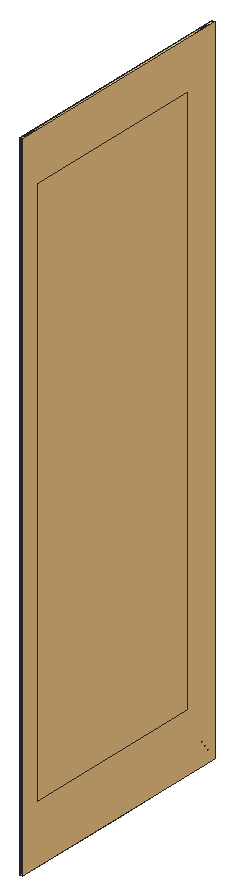
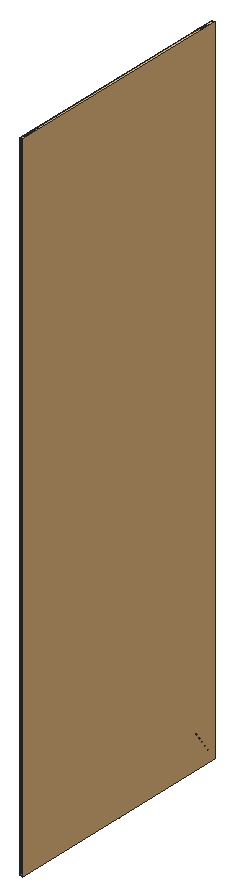
# SketchUp Ruby script. Lengths in inches.
U = 1.inch
M = Sketchup.active_model
def pt(a) = Geom::Point3d.new(a.map { |v| v * U })
def face(e, loops, mat)
  f = e.add_face(loops[0].map { |a| pt(a) })
  loops[1..].each { |l| e.add_face(l.map { |a| pt(a) }).erase! }
  f.material = f.back_material = mat if mat
  f
end
# faces: each face lists its corners as indices into pts; further lists are holes
def faces(e, pts, list, mat = nil) = list.each { |f| face(e, (f[0].is_a?(Array) ? f : [f]).map { |l| l.map { |i| pts[i] } }, mat) }
# xy, xz, yz: faces in a plane at the given z, y or x. An outline is a flat list of corners, or four numbers for a rectangle; further outlines are holes
def ring(l) = l.size == 4 ? [[l[0], l[1]], [l[2], l[1]], [l[2], l[3]], [l[0], l[3]]] : l.each_slice(2).to_a
def flat(e, list, mat, &to3) = list.each { |f| face(e, (f[0].is_a?(Array) ? f : [f]).map { |l| ring(l).map { |u, v| to3.(u, v) } }, mat) }
def xy(e, z, list, mat = nil) = flat(e, list, mat) { |x, y| [x, y, z] }
def xz(e, y, list, mat = nil) = flat(e, list, mat) { |x, z| [x, y, z] }
def yz(e, x, list, mat = nil) = flat(e, list, mat) { |y, z| [x, y, z] }
def lines(e, pts, list) = list.each { |a, b| e.add_line(pt(pts[a]), pt(pts[b])) }
# prism: a flat outline (further loops are holes) pulled along v
def prism(e, loops, v, mat = nil)
  f = face(e, loops, mat); d = Geom::Vector3d.new(v.map { |x| x * U })
  f.pushpull(f.normal.samedirection?(d) ? d.length : -d.length)
end
def box(e, o, s, mat = nil) = prism(e, [[o, [o[0] + s[0], o[1], o[2]], [o[0] + s[0], o[1] + s[1], o[2]], [o[0], o[1] + s[1], o[2]]]], [0, 0, s[2]], mat)
def at(x, y, z, deg = 0) = Geom::Transformation.translation(pt([x, y, z])) * Geom::Transformation.rotation(ORIGIN, Z_AXIS, deg.degrees)
def axes(o, x, y, z) = Geom::Transformation.new([*x, 0, *y, 0, *z, 0, *pt(o).to_a, 1])
def part(name) = M.definitions.add(name)
# library, detail: a bought-in or finely detailed component or shape, given as its bounding box
def library(name, o, s) = part(name).tap { |d| box(d.entities, o, s) }
def detail(e, o, s) = box(e.add_group.entities, o, s)
def put(e, d, t, mat = nil) = e.add_instance(d, t).tap { |i| i.material = mat if mat }
def group(e, t, mat = nil) = e.add_group.tap { |g| g.transformation = t; g.material = mat if mat }.entities
root = M.entities
M.materials.add("Material \#0").color = [86, 53, 35]
M.materials.add("Material \#1").color = [140, 140, 140]
c1 = part("3DGeom~8_Defintion")
xz(c1.entities,-471.94,[[458.125,-17.29,459.53,-16.11,457.73,-17.15],[458.125,-17.29,458.54,-17.29,459.53,-16.11],[458.54,-17.29,458.93,-17.15,459.53,-16.11],[457.73,-17.15,459.53,-16.11,457.42,-16.88],[458.93,-17.15,459.25,-16.88,459.53,-16.11],
  [457.42,-16.88,459.53,-16.11,457.21,-16.52],[459.25,-16.88,459.46,-16.52,459.53,-16.11],[457.21,-16.52,459.53,-16.11,457.14,-16.11],[457.14,-16.11,459.53,-16.11,457.21,-15.7],[459.53,-16.11,457.42,-15.34,457.21,-15.7],
  [459.53,-16.11,457.73,-15.07,457.42,-15.34],[459.53,-16.11,458.125,-14.93,457.73,-15.07],[459.53,-16.11,458.54,-14.93,458.125,-14.93],[459.53,-16.11,458.93,-15.07,458.54,-14.93],[459.53,-16.11,459.25,-15.34,458.93,-15.07],
  [459.53,-16.11,459.46,-15.7,459.25,-15.34]],"Material \#1")
xz(c1.entities,-416.39,[[458.125,-17.29,457.73,-17.15,459.53,-16.11],[458.125,-17.29,459.53,-16.11,458.54,-17.29],[458.54,-17.29,459.53,-16.11,458.93,-17.15],[457.73,-17.15,457.42,-16.88,459.53,-16.11],[458.93,-17.15,459.53,-16.11,459.25,-16.88],
  [457.42,-16.88,457.21,-16.52,459.53,-16.11],[459.25,-16.88,459.53,-16.11,459.46,-16.52],[457.21,-16.52,457.14,-16.11,459.53,-16.11],[457.14,-16.11,457.21,-15.7,459.53,-16.11],[459.53,-16.11,457.21,-15.7,457.42,-15.34],
  [459.53,-16.11,457.42,-15.34,457.73,-15.07],[459.53,-16.11,457.73,-15.07,458.125,-14.93],[459.53,-16.11,458.125,-14.93,458.54,-14.93],[459.53,-16.11,458.54,-14.93,458.93,-15.07],[459.53,-16.11,458.93,-15.07,459.25,-15.34],
  [459.53,-16.11,459.25,-15.34,459.46,-15.7]],"Material \#1")
xz(c1.entities,-27.5,[[458.125,-17.29,459.53,-16.11,457.73,-17.15],[458.125,-17.29,458.54,-17.29,459.53,-16.11],[458.54,-17.29,458.93,-17.15,459.53,-16.11],[457.73,-17.15,459.53,-16.11,457.42,-16.88],[458.93,-17.15,459.25,-16.88,459.53,-16.11],
  [457.42,-16.88,459.53,-16.11,457.21,-16.52],[459.25,-16.88,459.46,-16.52,459.53,-16.11],[457.21,-16.52,459.53,-16.11,457.14,-16.11],[457.14,-16.11,459.53,-16.11,457.21,-15.7],[459.53,-16.11,457.42,-15.34,457.21,-15.7],
  [459.53,-16.11,457.73,-15.07,457.42,-15.34],[459.53,-16.11,458.125,-14.93,457.73,-15.07],[459.53,-16.11,458.54,-14.93,458.125,-14.93],[459.53,-16.11,458.93,-15.07,458.54,-14.93],[459.53,-16.11,459.25,-15.34,458.93,-15.07],
  [459.53,-16.11,459.46,-15.7,459.25,-15.34]],"Material \#1")
xz(c1.entities,28.06,[[458.125,-17.29,457.73,-17.15,459.53,-16.11],[458.125,-17.29,459.53,-16.11,458.54,-17.29],[458.54,-17.29,459.53,-16.11,458.93,-17.15],[457.73,-17.15,457.42,-16.88,459.53,-16.11],[458.93,-17.15,459.53,-16.11,459.25,-16.88],
  [457.42,-16.88,457.21,-16.52,459.53,-16.11],[459.25,-16.88,459.53,-16.11,459.46,-16.52],[457.21,-16.52,457.14,-16.11,459.53,-16.11],[457.14,-16.11,457.21,-15.7,459.53,-16.11],[459.53,-16.11,457.21,-15.7,457.42,-15.34],
  [459.53,-16.11,457.42,-15.34,457.73,-15.07],[459.53,-16.11,457.73,-15.07,458.125,-14.93],[459.53,-16.11,458.125,-14.93,458.54,-14.93],[459.53,-16.11,458.54,-14.93,458.93,-15.07],[459.53,-16.11,458.93,-15.07,459.25,-15.34],
  [459.53,-16.11,459.25,-15.34,459.46,-15.7]],"Material \#1")
xz(c1.entities,472.5,[[458.125,-17.29,459.53,-16.11,457.73,-17.15],[458.125,-17.29,458.54,-17.29,459.53,-16.11],[458.54,-17.29,458.93,-17.15,459.53,-16.11],[457.73,-17.15,459.53,-16.11,457.42,-16.88],[458.93,-17.15,459.25,-16.88,459.53,-16.11],
  [457.42,-16.88,459.53,-16.11,457.21,-16.52],[459.25,-16.88,459.46,-16.52,459.53,-16.11],[457.21,-16.52,459.53,-16.11,457.14,-16.11],[457.14,-16.11,459.53,-16.11,457.21,-15.7],[459.53,-16.11,457.42,-15.34,457.21,-15.7],
  [459.53,-16.11,457.73,-15.07,457.42,-15.34],[459.53,-16.11,458.125,-14.93,457.73,-15.07],[459.53,-16.11,458.54,-14.93,458.125,-14.93],[459.53,-16.11,458.93,-15.07,458.54,-14.93],[459.53,-16.11,459.25,-15.34,458.93,-15.07],
  [459.53,-16.11,459.46,-15.7,459.25,-15.34]],"Material \#1")
xz(c1.entities,528.06,[[458.125,-17.29,457.73,-17.15,459.53,-16.11],[458.125,-17.29,459.53,-16.11,458.54,-17.29],[458.54,-17.29,459.53,-16.11,458.93,-17.15],[457.73,-17.15,457.42,-16.88,459.53,-16.11],[458.93,-17.15,459.53,-16.11,459.25,-16.88],
  [457.42,-16.88,457.21,-16.52,459.53,-16.11],[459.25,-16.88,459.53,-16.11,459.46,-16.52],[457.21,-16.52,457.14,-16.11,459.53,-16.11],[457.14,-16.11,457.21,-15.7,459.53,-16.11],[459.53,-16.11,457.21,-15.7,457.42,-15.34],
  [459.53,-16.11,457.42,-15.34,457.73,-15.07],[459.53,-16.11,457.73,-15.07,458.125,-14.93],[459.53,-16.11,458.125,-14.93,458.54,-14.93],[459.53,-16.11,458.54,-14.93,458.93,-15.07],[459.53,-16.11,458.93,-15.07,459.25,-15.34],
  [459.53,-16.11,459.25,-15.34,459.46,-15.7]],"Material \#1")
c2 = library("3DGeom~7_Defintion",[455.56,-471.94,-18.85],[5.55,1000,5.48])
c3 = library("3DGeom~9_Defintion",[456.52,-471.89,-18.89],[5.57,1000,5.49])
c4 = library("3DGeom~6_Defintion",[-5.59,-471.8,-48.03],[468.87,1000,73.72])
c5 = library("3DGeom~16_Defintion",[-962.62,-252.34,-11.22],[1000,504.68,93.46])
c6 = part("3DGeom~15_Defintion")
xy(c6.entities,0,[[-961.58,-251.9,-958.5,-248.8125,-961.58,-237.8],[-961.58,-251.9,28.8,-248.8125,-958.5,-248.8125],[-961.58,-251.9,36.25,-251.9,28.8,-248.8125],[36.25,-251.9,19.98,-239.99,28.8,-248.8125],[36.25,-251.9,22.16,-237.8,19.98,-239.99],
  [-958.5,-248.8125,-958.5,-237.8,-961.58,-237.8],[19.98,-239.99,22.16,-237.8,3.36,-223.37],[-958.5,-237.8,-958.5,-223.37,-961.58,-220.28],[-961.58,-237.8,-958.5,-237.8,-961.58,-220.28],[22.16,-237.8,4.64,-220.28,3.36,-223.37],
  [-958.5,-223.37,4.64,-220.28,-961.58,-220.28],[-958.5,-223.37,3.36,-223.37,4.64,-220.28],[5.29,-219.63,8.375,-218.35,5.29,0],[8.375,-218.35,8.375,0,5.29,0],[5.29,0,8.375,0,5.29,219.63],
  [8.375,0,8.375,218.35,5.29,219.63],[8.375,218.35,22.8125,237.15,5.29,219.63],[-961.58,220.28,-958.5,223.37,-961.58,237.8],[-961.58,220.28,3.36,223.37,-958.5,223.37],[-961.58,220.28,4.64,220.28,3.36,223.37],
  [4.64,220.28,19.98,239.99,3.36,223.37],[4.64,220.28,22.16,237.8,19.98,239.99],[-958.5,223.37,-958.5,237.8,-961.58,237.8],[-958.5,237.8,-958.5,248.8125,-961.58,251.9],[-961.58,237.8,-958.5,237.8,-961.58,251.9],
  [22.16,237.8,28.8,248.8125,19.98,239.99],[22.16,237.8,36.25,251.9,28.8,248.8125],[-958.5,248.8125,36.25,251.9,-961.58,251.9],[-958.5,248.8125,28.8,248.8125,36.25,251.9]],"Material \#0")
xy(c6.entities,7.48,[[-962.79,-238.36,23.37,-238.36,-962.79,-219.67],[23.37,-238.36,4.67,-219.67,-962.79,-219.67],[23.37,-238.36,23.37,0,4.67,-219.67],[4.67,-219.67,23.37,0,4.67,0],[23.37,0,23.37,238.36,4.67,219.67],
  [4.67,0,23.37,0,4.67,219.67],[-962.79,219.67,23.37,238.36,-962.79,238.36],[-962.79,219.67,4.67,219.67,23.37,238.36]],"Material \#0")
xy(c6.entities,63.5625,[[-962.79,-238.36,-962.79,-219.67,4.67,-219.67],[-962.79,-238.36,4.67,-219.67,23.37,-238.36],[23.37,-238.36,4.67,-219.67,23.37,0],[4.67,-219.67,4.67,0,23.37,0],[23.37,0,4.67,219.67,23.37,238.36],
  [4.67,0,4.67,219.67,23.37,0],[-962.79,219.67,-962.79,238.36,4.67,219.67],[4.67,219.67,-962.79,238.36,23.37,238.36]],"Material \#0")
xy(c6.entities,69.64,[[-962.79,-219.62,4.63,-219.62,-962.79,-200.32],[4.63,-219.62,-14.68,-200.32,-962.79,-200.32],[4.63,-219.62,4.63,0,-14.68,-200.32],[-14.68,-200.32,4.63,0,-14.68,0],[-14.68,0,4.63,0,-14.68,200.32],
  [4.63,0,4.63,219.62,-14.68,200.32],[-962.79,200.32,-14.68,200.32,4.63,219.62],[-962.79,200.32,4.63,219.62,-962.79,219.62]],"Material \#0")
xy(c6.entities,71.04,[[-961.58,-251.9,-958.5,-248.8125,28.8,-248.8125],[-961.58,-251.9,-961.58,-237.8,-958.5,-248.8125],[-961.58,-251.9,28.8,-248.8125,36.25,-251.9],[36.25,-251.9,19.98,-239.99,22.16,-237.8],[36.25,-251.9,28.8,-248.8125,19.98,-239.99],
  [-958.5,-248.8125,-961.58,-237.8,-958.5,-237.8],[19.98,-239.99,3.36,-223.37,22.16,-237.8],[-958.5,-237.8,-961.58,-220.28,-958.5,-223.37],[-961.58,-237.8,-961.58,-220.28,-958.5,-237.8],[22.16,-237.8,3.36,-223.37,4.64,-220.28],
  [-958.5,-223.37,-961.58,-220.28,4.64,-220.28],[-958.5,-223.37,4.64,-220.28,3.36,-223.37],[5.29,-219.63,5.29,0,8.375,-218.35],[8.375,-218.35,5.29,0,8.375,0],[5.29,0,5.29,219.63,8.375,0],
  [8.375,0,5.29,219.63,8.375,218.35],[8.375,218.35,5.29,219.63,22.8125,237.15],[-961.58,220.28,-958.5,223.37,3.36,223.37],[-961.58,220.28,-961.58,237.8,-958.5,223.37],[-961.58,220.28,3.36,223.37,4.64,220.28],
  [4.64,220.28,3.36,223.37,19.98,239.99],[4.64,220.28,19.98,239.99,22.16,237.8],[-958.5,223.37,-961.58,237.8,-958.5,237.8],[-958.5,237.8,-961.58,251.9,-958.5,248.8125],[-961.58,237.8,-961.58,251.9,-958.5,237.8],
  [22.16,237.8,19.98,239.99,28.8,248.8125],[22.16,237.8,28.8,248.8125,36.25,251.9],[-958.5,248.8125,-961.58,251.9,36.25,251.9],[-958.5,248.8125,36.25,251.9,28.8,248.8125]],"Material \#0")
xz(c6.entities,-238.36,[[-962.79,63.5625,23.37,63.5625,23.37,72.07],[-962.79,63.5625,23.37,72.07,-962.79,72.07]],"Material \#0")
xz(c6.entities,-219.67,[[-962.79,7.48,4.67,7.48,-962.79,63.5625],[4.67,7.48,4.67,63.5625,-962.79,63.5625]],"Material \#0")
xz(c6.entities,219.67,[[-962.79,7.48,-962.79,63.5625,4.67,7.48],[4.67,7.48,-962.79,63.5625,4.67,63.5625]],"Material \#0")
xz(c6.entities,238.36,[[-962.79,63.5625,-962.79,72.07,23.37,72.07],[-962.79,63.5625,23.37,72.07,23.37,63.5625]],"Material \#0")
yz(c6.entities,4.67,[[-219.67,7.48,0,7.48,-219.67,63.5625],[0,7.48,0,63.5625,-219.67,63.5625],[0,7.48,219.67,63.5625,0,63.5625],[0,7.48,219.67,7.48,219.67,63.5625]],"Material \#0")
yz(c6.entities,23.37,[[-238.36,63.5625,0,63.5625,-238.36,72.07],[0,63.5625,0,72.07,-238.36,72.07],[0,63.5625,238.36,63.5625,238.36,72.07],[0,63.5625,238.36,72.07,0,72.07]],"Material \#0")
p = [[36.9,-251.24,0],[37.21,0,-0.16],[34.125,0,-0.14],[36.9,251.24,0],[33.83,243.81,0.02],[33.83,-243.8,0.02],
  [22.8125,-237.15,0],[24.99,-234.97,-0.01],[5.375,-220.37,0],[23.37,-238.36,7.48],[4.67,-219.67,7.48],[4.67,-219.67,7.48],
  [23.37,-238.36,7.48],[23.37,-238.36,0],[4.67,-219.67,7.48],[23.37,-238.36,0],[5.375,-220.37,0],[5.375,-220.37,0],
  [23.37,-238.36,0],[5.29,-219.63,0],[8.375,-218.35,0],[-15.36,-199.64,1.62],[4.67,-219.67,7.48],[5.375,-220.37,0],
  [-13.8,-201.19,0.06],[5.375,-220.37,0],[5.375,-220.37,0],[-14.84,-200.15,0.58],[5.375,-220.37,0],[-13.8,-201.19,0.06],
  [-6.08,-208.92,0],[5.375,-220.37,0],[-13.8,-201.19,0.06],[-6.08,-208.92,0],[-13.8,-201.19,0.06],[5.375,-220.37,0],
  [-6.08,-208.92,0],[-13.8,-201.19,0.06],[-13.09,-201.91,0],[-6.08,-208.92,0],[-13.09,-201.91,0],[-13.8,-201.19,0.06],
  [-15.36,199.64,1.62],[4.67,219.67,7.48],[5.375,220.37,0],[-13.8,201.19,0.06],[5.375,220.37,0],[5.375,220.37,0],
  [4.67,219.67,7.48],[-14.84,200.15,0.58],[5.375,220.37,0],[-13.8,201.19,0.06],[-6.08,208.92,0],[-13.09,201.91,0],
  [-13.8,201.19,0.06],[-6.08,208.92,0],[-13.8,201.19,0.06],[5.375,220.37,0],[-6.08,208.92,0],[5.375,220.37,0],
  [-13.8,201.19,0.06],[-6.08,208.92,0],[-13.8,201.19,0.06],[-13.09,201.91,0],[8.375,218.35,0],[24.99,234.97,-0.01],
  [22.8125,237.15,0],[23.37,238.36,7.48],[23.37,238.36,0],[23.37,238.36,0],[5.375,220.37,0],[5.375,220.37,0],
  [23.37,238.36,7.48],[4.67,219.67,7.48],[5.375,220.37,0],[23.37,238.36,0],[23.37,238.36,7.48],[-13.8,-201.19,0.06],
  [-14.84,-200.15,0.58],[-14.38,-200.61,0.26],[-13.8,-201.19,0.06],[-13.8,-201.19,0.06],[-14.38,-200.61,0.26],[-13.8,201.19,0.06],
  [-14.84,200.15,0.58],[-13.8,201.19,0.06],[-14.38,200.61,0.26],[-14.38,200.61,0.26],[-13.8,201.19,0.06],[4.63,-219.62,69.64],
  [4.63,-219.62,69.64],[-15.42,-199.57,9.43],[-15.36,-199.64,1.62],[-15.16,-199.83,1.04],[-15.16,-199.83,1.04],[-15.16,199.83,1.04],
  [-15.36,199.64,1.62],[-15.16,199.83,1.04],[-15.42,199.57,9.43],[4.63,219.62,69.64],[4.67,219.67,7.48],[4.63,219.62,69.64],
  [4.63,-219.62,69.64],[4.67,-219.67,63.5625],[4.67,-219.67,63.5625],[4.67,-219.67,7.48],[-15.28,-199.71,69.25],[4.63,-219.62,69.64],
  [-15.42,-199.57,9.43],[-15.28,-199.71,69.25],[-15.42,-199.57,2.34],[-15.42,-199.57,2.34],[-15.42,199.57,2.34],[-15.42,199.57,9.43],
  [-15.28,199.71,69.25],[-15.28,199.71,69.25],[4.63,219.62,69.64],[4.63,219.62,69.64],[4.67,219.67,63.5625],[4.67,219.67,63.5625],
  [-15.42,199.57,2.34],[4.67,-219.67,63.5625],[4.63,-219.62,69.64],[4.67,219.67,7.48],[4.67,219.67,63.5625],[4.63,219.62,69.64],
  [4.63,-219.62,69.64],[-15.28,-199.71,69.25],[-15.28,-199.71,69.25],[-15.42,-199.57,48.99],[-15.42,-199.57,48.99],[-15.28,-199.71,69.25],
  [-15.42,199.57,48.99],[-15.28,199.71,69.25],[-15.28,199.71,69.25],[-15.42,199.57,48.99],[4.63,219.62,69.64],[4.63,-219.62,69.64],
  [23.37,-238.36,72.07],[4.67,-219.67,63.5625],[4.67,-219.67,63.5625],[23.37,-238.36,63.5625],[23.37,-238.36,72.07],[4.67,-219.67,63.5625],
  [5.24,-220.23,70.03],[23.37,-238.36,72.07],[23.37,-238.36,63.5625],[4.67,-219.67,63.5625],[4.67,-219.67,63.5625],[4.63,-219.62,69.64],
  [4.63,219.62,69.64],[23.37,238.36,72.07],[4.67,219.67,63.5625],[4.67,219.67,63.5625],[5.24,220.23,70.03],[4.63,219.62,69.64],
  [23.37,238.36,63.5625],[4.67,219.67,63.5625],[4.67,219.67,63.5625],[23.37,238.36,63.5625],[23.37,238.36,72.07],[4.67,219.67,63.5625],
  [23.37,238.36,72.07],[4.63,-219.62,69.64],[-14.68,-200.32,69.64],[-15.28,-199.71,69.25],[-15.28,-199.71,69.25],[-14.68,-200.32,69.64],
  [4.63,-219.62,69.64],[-15.28,199.71,69.25],[-14.68,200.32,69.64],[4.63,219.62,69.64],[4.63,219.62,69.64],[-14.68,200.32,69.64],
  [4.63,-219.62,69.64],[5.24,-220.23,70.03],[23.37,-238.36,72.07],[4.63,219.62,69.64],[5.24,220.23,70.03],[5.375,-220.37,72.07],
  [5.375,-220.37,72.07],[23.37,-238.36,72.07],[5.375,220.37,72.07],[23.37,238.36,72.07],[5.375,220.37,72.07],[33.83,-243.8,71.03],
  [36.9,-251.24,71.04],[22.8125,-237.15,71.04],[34.125,0,71.19],[37.21,0,71.2],[24.99,-234.97,71.05],[5.29,-219.63,71.04],
  [8.375,-218.35,71.04],[33.83,243.81,71.03],[36.9,251.24,71.04],[22.8125,237.15,71.04],[24.99,234.97,71.05],[8.375,218.35,71.04]]
faces(c6.entities,p,[[0,1,2],[1,3,4],[4,2,1],[2,5,0],[6,0,5],[5,7,6],[8,9,10],[11,12,13],
  [14,15,16],[17,18,9],[19,6,7],[7,20,19],[21,22,23],[24,21,25],[26,10,27],[28,27,29],
  [30,31,32],[33,34,35],[36,37,38],[39,40,41],[42,43,44],[45,42,46],[47,48,49],[50,49,51],
  [52,53,54],[55,56,57],[58,59,60],[61,62,63],[64,65,66],[43,67,68],[43,69,70],[71,72,73],
  [74,75,76],[3,66,65],[65,4,3],[77,78,21],[27,79,80],[81,82,78],[83,84,42],[85,86,84],
  [49,87,88],[10,89,27],[90,91,27],[92,93,27],[91,92,27],[78,94,21],[84,95,42],[96,97,49],
  [98,96,49],[99,98,49],[100,101,49],[21,102,103],[21,104,105],[21,106,107],[21,108,109],[91,110,92],
  [21,111,108],[42,112,113],[42,113,114],[42,115,116],[42,117,118],[42,119,43],[98,120,96],[10,121,122],
  [123,124,125],[126,127,91],[128,129,91],[108,130,131],[113,132,133],[134,135,98],[136,134,98],[137,138,139],
  [140,141,142],[143,142,144],[145,146,147],[148,144,149],[150,151,152],[153,154,155],[151,156,157],[158,159,160],
  [161,162,154],[163,164,165],[166,167,168],[169,170,171],[172,173,134],[174,175,176],[177,178,151],[142,179,144],
  [175,180,181],[178,182,151],[183,184,154],[185,186,187],[186,185,188],[188,189,186],[187,190,185],[190,187,191],
  [191,192,190],[189,188,193],[193,194,189],[195,196,197],[196,195,194],[194,193,196]],"Material \#0")
xy(root,8.271,[[155.733,414.099,155.728,414.11,155.733,414.117],[155.733,414.099,155.733,414.117,155.737,414.127],[155.733,414.099,155.737,414.127,155.737,414.11],[155.728,414.11,155.725,414.141,155.729,414.127],[155.728,414.11,155.729,414.127,155.733,414.117],
  [155.737,414.11,155.737,414.127,155.74,414.155],[155.737,414.11,155.74,414.155,155.741,414.141],[155.729,414.127,155.725,414.141,155.725,414.155],[155.725,414.141,155.722,414.189,155.725,414.155],[155.741,414.141,155.74,414.155,155.742,414.198],
  [155.741,414.141,155.742,414.198,155.744,414.189],[155.725,414.155,155.722,414.189,155.723,414.198],[155.722,414.189,155.72,414.248,155.723,414.198],[155.744,414.189,155.742,414.198,155.744,414.251],[155.744,414.189,155.744,414.251,155.745,414.248],
  [155.723,414.198,155.72,414.248,155.721,414.251],[155.72,414.248,155.72,414.311,155.721,414.251],[155.745,414.248,155.744,414.251,155.744,414.308],[155.745,414.248,155.744,414.308,155.745,414.311],[155.721,414.251,155.72,414.311,155.721,414.308],
  [155.721,414.308,155.72,414.311,155.722,414.37],[155.721,414.308,155.722,414.37,155.723,414.361],[155.744,414.308,155.742,414.361,155.745,414.311],[155.745,414.311,155.742,414.361,155.744,414.37],[155.723,414.361,155.722,414.37,155.725,414.417],
  [155.723,414.361,155.725,414.417,155.725,414.404],[155.742,414.361,155.74,414.404,155.744,414.37],[155.744,414.37,155.74,414.404,155.741,414.417],[155.725,414.404,155.725,414.417,155.728,414.449],[155.725,414.404,155.728,414.449,155.729,414.432],
  [155.74,414.404,155.737,414.432,155.741,414.417],[155.741,414.417,155.737,414.432,155.737,414.449],[155.729,414.432,155.728,414.449,155.733,414.46],[155.729,414.432,155.733,414.46,155.733,414.442],[155.737,414.432,155.733,414.442,155.737,414.449],
  [155.733,414.442,155.733,414.46,155.737,414.449]],"Material \#1")
xy(root,8.291,[[155.733,414.099,155.729,414.127,155.728,414.11],[155.733,414.099,155.733,414.117,155.729,414.127],[155.733,414.099,155.737,414.11,155.733,414.117],[155.728,414.11,155.725,414.155,155.725,414.141],[155.728,414.11,155.729,414.127,155.725,414.155],
  [155.737,414.11,155.737,414.127,155.733,414.117],[155.737,414.11,155.741,414.141,155.737,414.127],[155.737,414.127,155.741,414.141,155.74,414.155],[155.725,414.141,155.723,414.198,155.722,414.189],[155.725,414.141,155.725,414.155,155.723,414.198],
  [155.741,414.141,155.744,414.189,155.74,414.155],[155.74,414.155,155.744,414.189,155.742,414.198],[155.722,414.189,155.721,414.251,155.72,414.248],[155.722,414.189,155.723,414.198,155.721,414.251],[155.744,414.189,155.745,414.248,155.742,414.198],
  [155.742,414.198,155.745,414.248,155.744,414.251],[155.72,414.248,155.721,414.251,155.721,414.308],[155.72,414.248,155.721,414.308,155.72,414.311],[155.745,414.248,155.745,414.311,155.744,414.251],[155.744,414.251,155.745,414.311,155.744,414.308],
  [155.721,414.308,155.723,414.361,155.72,414.311],[155.744,414.308,155.744,414.37,155.742,414.361],[155.744,414.308,155.745,414.311,155.744,414.37],[155.72,414.311,155.723,414.361,155.722,414.37],[155.723,414.361,155.725,414.404,155.722,414.37],
  [155.742,414.361,155.741,414.417,155.74,414.404],[155.742,414.361,155.744,414.37,155.741,414.417],[155.722,414.37,155.725,414.404,155.725,414.417],[155.725,414.404,155.729,414.432,155.725,414.417],[155.74,414.404,155.737,414.449,155.737,414.432],
  [155.74,414.404,155.741,414.417,155.737,414.449],[155.725,414.417,155.729,414.432,155.728,414.449],[155.729,414.432,155.733,414.442,155.728,414.449],[155.737,414.432,155.733,414.46,155.733,414.442],[155.737,414.432,155.737,414.449,155.733,414.46],
  [155.733,414.442,155.733,414.46,155.728,414.449]],"Material \#1")
xy(root,12.796,[[155.733,414.099,155.728,414.11,155.729,414.127],[155.733,414.099,155.729,414.127,155.733,414.117],[155.733,414.099,155.733,414.117,155.737,414.11],[155.728,414.11,155.725,414.141,155.725,414.155],[155.728,414.11,155.725,414.155,155.729,414.127],
  [155.737,414.11,155.733,414.117,155.737,414.127],[155.737,414.11,155.737,414.127,155.741,414.141],[155.737,414.127,155.74,414.155,155.741,414.141],[155.725,414.141,155.722,414.189,155.723,414.198],[155.725,414.141,155.723,414.198,155.725,414.155],
  [155.741,414.141,155.74,414.155,155.744,414.189],[155.74,414.155,155.742,414.198,155.744,414.189],[155.722,414.189,155.72,414.248,155.721,414.251],[155.722,414.189,155.721,414.251,155.723,414.198],[155.744,414.189,155.742,414.198,155.745,414.248],
  [155.742,414.198,155.744,414.251,155.745,414.248],[155.72,414.248,155.72,414.311,155.721,414.308],[155.72,414.248,155.721,414.308,155.721,414.251],[155.745,414.248,155.744,414.251,155.745,414.311],[155.744,414.251,155.744,414.308,155.745,414.311],
  [155.721,414.308,155.72,414.311,155.723,414.361],[155.744,414.308,155.742,414.361,155.744,414.37],[155.744,414.308,155.744,414.37,155.745,414.311],[155.72,414.311,155.722,414.37,155.723,414.361],[155.723,414.361,155.722,414.37,155.725,414.404],
  [155.742,414.361,155.74,414.404,155.741,414.417],[155.742,414.361,155.741,414.417,155.744,414.37],[155.722,414.37,155.725,414.417,155.725,414.404],[155.725,414.404,155.725,414.417,155.729,414.432],[155.74,414.404,155.737,414.432,155.737,414.449],
  [155.74,414.404,155.737,414.449,155.741,414.417],[155.725,414.417,155.728,414.449,155.729,414.432],[155.729,414.432,155.728,414.449,155.733,414.442],[155.737,414.432,155.733,414.442,155.733,414.46],[155.737,414.432,155.733,414.46,155.737,414.449],
  [155.733,414.442,155.728,414.449,155.733,414.46]],"Material \#1")
xy(root,12.816,[[155.733,414.099,155.733,414.117,155.728,414.11],[155.733,414.099,155.737,414.11,155.737,414.127],[155.733,414.099,155.737,414.127,155.733,414.117],[155.728,414.11,155.729,414.127,155.725,414.141],[155.728,414.11,155.733,414.117,155.729,414.127],
  [155.737,414.11,155.74,414.155,155.737,414.127],[155.737,414.11,155.741,414.141,155.74,414.155],[155.729,414.127,155.725,414.155,155.725,414.141],[155.725,414.141,155.725,414.155,155.722,414.189],[155.741,414.141,155.742,414.198,155.74,414.155],
  [155.741,414.141,155.744,414.189,155.742,414.198],[155.725,414.155,155.723,414.198,155.722,414.189],[155.722,414.189,155.723,414.198,155.72,414.248],[155.744,414.189,155.744,414.251,155.742,414.198],[155.744,414.189,155.745,414.248,155.744,414.251],
  [155.723,414.198,155.721,414.251,155.72,414.248],[155.72,414.248,155.721,414.251,155.72,414.311],[155.745,414.248,155.744,414.308,155.744,414.251],[155.745,414.248,155.745,414.311,155.744,414.308],[155.721,414.251,155.721,414.308,155.72,414.311],
  [155.721,414.308,155.722,414.37,155.72,414.311],[155.721,414.308,155.723,414.361,155.722,414.37],[155.744,414.308,155.745,414.311,155.742,414.361],[155.745,414.311,155.744,414.37,155.742,414.361],[155.723,414.361,155.725,414.417,155.722,414.37],
  [155.723,414.361,155.725,414.404,155.725,414.417],[155.742,414.361,155.744,414.37,155.74,414.404],[155.744,414.37,155.741,414.417,155.74,414.404],[155.725,414.404,155.728,414.449,155.725,414.417],[155.725,414.404,155.729,414.432,155.728,414.449],
  [155.74,414.404,155.741,414.417,155.737,414.432],[155.741,414.417,155.737,414.449,155.737,414.432],[155.729,414.432,155.733,414.46,155.728,414.449],[155.729,414.432,155.733,414.442,155.733,414.46],[155.737,414.432,155.737,414.449,155.733,414.442],
  [155.733,414.442,155.737,414.449,155.733,414.46]],"Material \#1")
xy(root,53.475,[[155.733,414.099,155.728,414.11,155.733,414.117],[155.733,414.099,155.733,414.117,155.737,414.127],[155.733,414.099,155.737,414.127,155.737,414.11],[155.728,414.11,155.725,414.141,155.729,414.127],[155.728,414.11,155.729,414.127,155.733,414.117],
  [155.737,414.11,155.737,414.127,155.74,414.155],[155.737,414.11,155.74,414.155,155.741,414.141],[155.729,414.127,155.725,414.141,155.725,414.155],[155.725,414.141,155.722,414.189,155.725,414.155],[155.741,414.141,155.74,414.155,155.742,414.198],
  [155.741,414.141,155.742,414.198,155.744,414.189],[155.725,414.155,155.722,414.189,155.723,414.198],[155.722,414.189,155.72,414.248,155.723,414.198],[155.744,414.189,155.742,414.198,155.744,414.251],[155.744,414.189,155.744,414.251,155.745,414.248],
  [155.723,414.198,155.72,414.248,155.721,414.251],[155.72,414.248,155.72,414.311,155.721,414.251],[155.745,414.248,155.744,414.251,155.744,414.308],[155.745,414.248,155.744,414.308,155.745,414.311],[155.721,414.251,155.72,414.311,155.721,414.308],
  [155.721,414.308,155.72,414.311,155.722,414.37],[155.721,414.308,155.722,414.37,155.723,414.361],[155.744,414.308,155.742,414.361,155.745,414.311],[155.745,414.311,155.742,414.361,155.744,414.37],[155.723,414.361,155.722,414.37,155.725,414.417],
  [155.723,414.361,155.725,414.417,155.725,414.404],[155.742,414.361,155.74,414.404,155.744,414.37],[155.744,414.37,155.74,414.404,155.741,414.417],[155.725,414.404,155.725,414.417,155.728,414.449],[155.725,414.404,155.728,414.449,155.729,414.432],
  [155.74,414.404,155.737,414.432,155.741,414.417],[155.741,414.417,155.737,414.432,155.737,414.449],[155.729,414.432,155.728,414.449,155.733,414.46],[155.729,414.432,155.733,414.46,155.733,414.442],[155.737,414.432,155.733,414.442,155.737,414.449],
  [155.733,414.442,155.733,414.46,155.737,414.449]],"Material \#1")
xy(root,53.495,[[155.733,414.099,155.729,414.127,155.728,414.11],[155.733,414.099,155.733,414.117,155.729,414.127],[155.733,414.099,155.737,414.11,155.733,414.117],[155.728,414.11,155.725,414.155,155.725,414.141],[155.728,414.11,155.729,414.127,155.725,414.155],
  [155.737,414.11,155.737,414.127,155.733,414.117],[155.737,414.11,155.741,414.141,155.737,414.127],[155.737,414.127,155.741,414.141,155.74,414.155],[155.725,414.141,155.723,414.198,155.722,414.189],[155.725,414.141,155.725,414.155,155.723,414.198],
  [155.741,414.141,155.744,414.189,155.74,414.155],[155.74,414.155,155.744,414.189,155.742,414.198],[155.722,414.189,155.721,414.251,155.72,414.248],[155.722,414.189,155.723,414.198,155.721,414.251],[155.744,414.189,155.745,414.248,155.742,414.198],
  [155.742,414.198,155.745,414.248,155.744,414.251],[155.72,414.248,155.721,414.251,155.721,414.308],[155.72,414.248,155.721,414.308,155.72,414.311],[155.745,414.248,155.745,414.311,155.744,414.251],[155.744,414.251,155.745,414.311,155.744,414.308],
  [155.721,414.308,155.723,414.361,155.72,414.311],[155.744,414.308,155.744,414.37,155.742,414.361],[155.744,414.308,155.745,414.311,155.744,414.37],[155.72,414.311,155.723,414.361,155.722,414.37],[155.723,414.361,155.725,414.404,155.722,414.37],
  [155.742,414.361,155.741,414.417,155.74,414.404],[155.742,414.361,155.744,414.37,155.741,414.417],[155.722,414.37,155.725,414.404,155.725,414.417],[155.725,414.404,155.729,414.432,155.725,414.417],[155.74,414.404,155.737,414.449,155.737,414.432],
  [155.74,414.404,155.741,414.417,155.737,414.449],[155.725,414.417,155.729,414.432,155.728,414.449],[155.729,414.432,155.733,414.442,155.728,414.449],[155.737,414.432,155.733,414.46,155.733,414.442],[155.737,414.432,155.737,414.449,155.733,414.46],
  [155.733,414.442,155.733,414.46,155.728,414.449]],"Material \#1")
put(root,c1,axes([155.66,444.02,55.77],[0,-0.0649,0],[0,0,-0.09041],[-0.00454,0,0]),"Material \#1")
put(root,c2,axes([155.66,444.02,55.77],[0,-0.0649,0],[0,0,-0.09041],[-0.00454,0,0]),"Material \#1")
put(root,c3,axes([155.66,444.02,55.77],[0,-0.06476,0],[0,0,-0.09022],[-0.00453,0,0]),"Material \#1")
put(root,c4,axes([155.66,444.02,55.77],[0,-0.06455,0],[0,0,-0.08993],[-0.00451,0,0]),"Material \#1")
put(root,c5,axes([155.34,430.68,2.53],[0,0,-0.10749],[0,-0.07715,0],[0.0054,0,0]),"Material \#0")
put(root,c6,axes([155.34,430.68,2.53],[0,0,-0.10747],[0,-0.07714,0],[0.00539,0,0]),"Material \#0")
